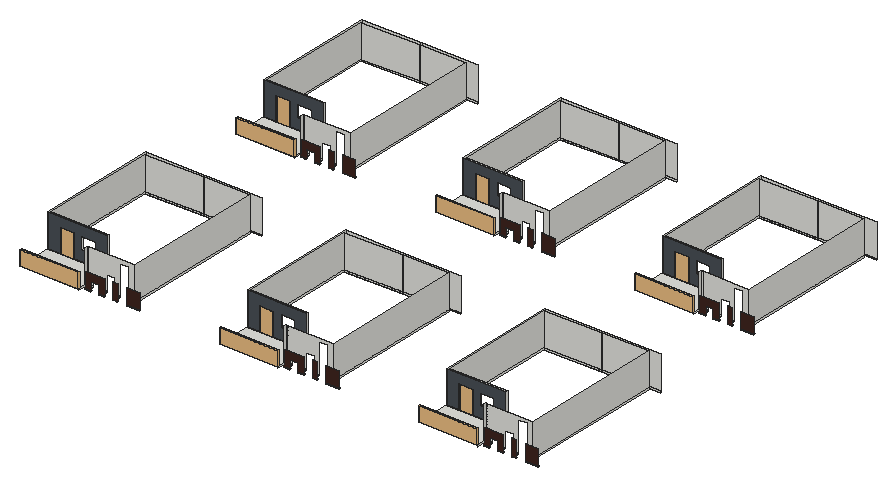
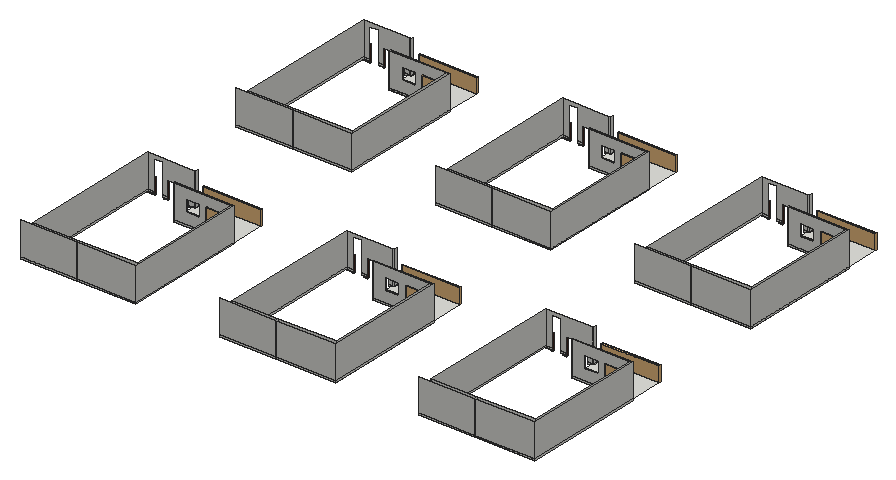
# SketchUp Ruby script. Lengths in inches.
U = 1.inch
M = Sketchup.active_model
def pt(a) = Geom::Point3d.new(a.map { |v| v * U })
def face(e, loops, mat)
  f = e.add_face(loops[0].map { |a| pt(a) })
  loops[1..].each { |l| e.add_face(l.map { |a| pt(a) }).erase! }
  f.material = f.back_material = mat if mat
  f
end
# faces: each face lists its corners as indices into pts; further lists are holes
def faces(e, pts, list, mat = nil) = list.each { |f| face(e, (f[0].is_a?(Array) ? f : [f]).map { |l| l.map { |i| pts[i] } }, mat) }
# xy, xz, yz: faces in a plane at the given z, y or x. An outline is a flat list of corners, or four numbers for a rectangle; further outlines are holes
def ring(l) = l.size == 4 ? [[l[0], l[1]], [l[2], l[1]], [l[2], l[3]], [l[0], l[3]]] : l.each_slice(2).to_a
def flat(e, list, mat, &to3) = list.each { |f| face(e, (f[0].is_a?(Array) ? f : [f]).map { |l| ring(l).map { |u, v| to3.(u, v) } }, mat) }
def xy(e, z, list, mat = nil) = flat(e, list, mat) { |x, y| [x, y, z] }
def xz(e, y, list, mat = nil) = flat(e, list, mat) { |x, z| [x, y, z] }
def yz(e, x, list, mat = nil) = flat(e, list, mat) { |y, z| [x, y, z] }
def lines(e, pts, list) = list.each { |a, b| e.add_line(pt(pts[a]), pt(pts[b])) }
# prism: a flat outline (further loops are holes) pulled along v
def prism(e, loops, v, mat = nil)
  f = face(e, loops, mat); d = Geom::Vector3d.new(v.map { |x| x * U })
  f.pushpull(f.normal.samedirection?(d) ? d.length : -d.length)
end
def box(e, o, s, mat = nil) = prism(e, [[o, [o[0] + s[0], o[1], o[2]], [o[0] + s[0], o[1] + s[1], o[2]], [o[0], o[1] + s[1], o[2]]]], [0, 0, s[2]], mat)
def at(x, y, z, deg = 0) = Geom::Transformation.translation(pt([x, y, z])) * Geom::Transformation.rotation(ORIGIN, Z_AXIS, deg.degrees)
def axes(o, x, y, z) = Geom::Transformation.new([*x, 0, *y, 0, *z, 0, *pt(o).to_a, 1])
def part(name) = M.definitions.add(name)
# library, detail: a bought-in or finely detailed component or shape, given as its bounding box
def library(name, o, s) = part(name).tap { |d| box(d.entities, o, s) }
def detail(e, o, s) = box(e.add_group.entities, o, s)
def put(e, d, t, mat = nil) = e.add_instance(d, t).tap { |i| i.material = mat if mat }
def group(e, t, mat = nil) = e.add_group.tap { |g| g.transformation = t; g.material = mat if mat }.entities
root = M.entities
M.materials.add("[0043_SaddleBrown]").color = [63, 38, 31]
M.materials.add("[Formica Blue]").color = [73, 80, 86]
c1 = library("Glass Railing",[0,0,0],[139.5,4.76,42])
c2 = library("door (1)",[38.93,25.48,0],[40,9.94,82.68])
xy(root,243.96,[[348.1875,438.72,370.54,441.04],[399.16,438.72,419.76,441.04],[451.01,438.72,467.3,441.04],[1072.625,438.72,1094.98,441.04],[1123.6,438.72,1144.2,441.04],
  [1175.45,438.72,1191.74,441.04],[1797.0625,438.72,1819.41,441.04],[1848.04,438.72,1868.64,441.04],[1899.89,438.72,1916.17,441.04],[500.42,438.73,547.05,441.04],
  [1224.86,438.73,1271.49,441.04],[1949.3,438.73,1995.93,441.04],[348.1875,1419.07,370.54,1421.39],[399.16,1419.07,419.76,1421.39],[451.01,1419.07,467.3,1421.39],
  [1072.625,1419.07,1094.98,1421.39],[1123.6,1419.07,1144.2,1421.39],[1175.45,1419.07,1191.74,1421.39],[1797.0625,1419.07,1819.41,1421.39],[1848.04,1419.07,1868.64,1421.39],
  [1899.89,1419.07,1916.17,1421.39],[500.42,1419.08,547.05,1421.39],[1224.86,1419.08,1271.49,1421.39],[1949.3,1419.08,1995.93,1421.39]])
xy(root,245.59,[[451.01,438.72,467.3,441.04],[1175.45,438.72,1191.74,441.04],[1899.89,438.72,1916.17,441.04],[451.01,1419.07,467.3,1421.39],[1175.45,1419.07,1191.74,1421.39],
  [1899.89,1419.07,1916.17,1421.39]])
xy(root,246.18,[[399.16,438.72,419.76,441.04],[1123.6,438.72,1144.2,441.04],[1848.04,438.72,1868.64,441.04],[399.16,1419.07,419.76,1421.39],[1123.6,1419.07,1144.2,1421.39],
  [1848.04,1419.07,1868.64,1421.39]])
xy(root,246.28,[[500.42,438.73,547.05,441.04],[1224.86,438.73,1271.49,441.04],[1949.3,438.73,1995.93,441.04],[500.42,1419.08,547.05,1421.39],[1224.86,1419.08,1271.49,1421.39],
  [1949.3,1419.08,1995.93,1421.39]])
xy(root,246.4375,[[348.1875,438.72,370.54,441.04],[1072.625,438.72,1094.98,441.04],[1797.0625,438.72,1819.41,441.04],[348.1875,1419.07,370.54,1421.39],[1072.625,1419.07,1094.98,1421.39],
  [1797.0625,1419.07,1819.41,1421.39]])
xy(root,252.25,[[137.5,535.375,137.5,980.35,353.97,980.35,353.97,971.23,144.84,965.96,144.84,540.48,353.97,540.48,353.97,535.375],[861.9375,535.375,861.9375,980.35,1078.41,980.35,1078.41,971.23,869.28,965.96,869.28,540.48,1078.41,540.48,1078.41,535.375],[1586.375,535.375,1586.375,980.35,1802.84,980.35,1802.84,971.23,1593.72,965.96,1593.72,540.48,1802.84,540.48,1802.84,535.375],[137.5,1515.73,137.5,1960.7,353.97,1960.7,353.97,1951.58,144.84,1946.3125,144.84,1520.83,353.97,1520.83,353.97,1515.73],[861.9375,1515.73,861.9375,1960.7,1078.41,1960.7,1078.41,1951.58,869.28,1946.3125,869.28,1520.83,1078.41,1520.83,1078.41,1515.73],
  [1586.375,1515.73,1586.375,1960.7,1802.84,1960.7,1802.84,1951.58,1593.72,1946.3125,1593.72,1520.83,1802.84,1520.83,1802.84,1515.73]])
xy(root,258.25,[[137.5,412.04,348.1875,412.04,348.1875,447.84,353.97,447.84,353.97,535.375,137.5,535.375],[861.9375,412.04,1072.625,412.04,1072.625,447.84,1078.41,447.84,1078.41,535.375,861.9375,535.375],[1586.375,412.04,1797.0625,412.04,1797.0625,447.84,1802.84,447.84,1802.84,535.375,1586.375,535.375],[137.5,535.375,137.5,980.35,353.97,980.35,353.97,971.23,144.84,965.96,144.84,540.48,183.3,540.48,183.3,535.375],[183.3,535.375,231.3,540.48],
  [231.3,535.375,353.97,540.48],[861.9375,535.375,861.9375,980.35,1078.41,980.35,1078.41,971.23,869.28,965.96,869.28,540.48,907.74,540.48,907.74,535.375],[907.74,535.375,955.74,540.48],[955.74,535.375,1078.41,540.48],[1586.375,535.375,1586.375,980.35,1802.84,980.35,1802.84,971.23,1593.72,965.96,1593.72,540.48,1632.17,540.48,1632.17,535.375],
  [1632.17,535.375,1680.17,540.48],[1680.17,535.375,1802.84,540.48],[137.5,1392.39,348.1875,1392.39,348.1875,1428.19,353.97,1428.19,353.97,1515.73,137.5,1515.73],[861.9375,1392.39,1072.625,1392.39,1072.625,1428.19,1078.41,1428.19,1078.41,1515.73,861.9375,1515.73],[1586.375,1392.39,1797.0625,1392.39,1797.0625,1428.19,1802.84,1428.19,1802.84,1515.73,1586.375,1515.73],
  [137.5,1515.73,137.5,1960.7,353.97,1960.7,353.97,1951.58,144.84,1946.3125,144.84,1520.83,183.3,1520.83,183.3,1515.73],[183.3,1515.73,231.3,1520.83],[231.3,1515.73,353.97,1520.83],[861.9375,1515.73,861.9375,1960.7,1078.41,1960.7,1078.41,1951.58,869.28,1946.3125,869.28,1520.83,907.74,1520.83,907.74,1515.73],[907.74,1515.73,955.74,1520.83],
  [955.74,1515.73,1078.41,1520.83],[1586.375,1515.73,1586.375,1960.7,1802.84,1960.7,1802.84,1951.58,1593.72,1946.3125,1593.72,1520.83,1632.17,1520.83,1632.17,1515.73],[1632.17,1515.73,1680.17,1520.83],[1680.17,1515.73,1802.84,1520.83]])
xy(root,275.89,[[370.54,438.72,399.16,447.84],[1094.98,438.72,1123.6,447.84],[1819.41,438.72,1848.04,447.84],[370.54,1419.07,399.16,1428.19],[1094.98,1419.07,1123.6,1428.19],
  [1819.41,1419.07,1848.04,1428.19]])
xz(root,438.72,[[451.01,245.59,467.3,303],[1175.45,245.59,1191.74,303],[1899.89,245.59,1916.17,303],[399.16,246.18,419.76,246.18,419.76,303,348.1875,303,348.1875,246.4375,370.54,246.4375,370.54,275.89,399.16,275.89],[1123.6,246.18,1144.2,246.18,1144.2,303,1072.625,303,1072.625,246.4375,1094.98,246.4375,1094.98,275.89,1123.6,275.89],
  [1848.04,246.18,1868.64,246.18,1868.64,303,1797.0625,303,1797.0625,246.4375,1819.41,246.4375,1819.41,275.89,1848.04,275.89]],"[0043_SaddleBrown]")
xz(root,438.73,[[500.42,246.28,547.05,303],[1224.86,246.28,1271.49,303],[1949.3,246.28,1995.93,303]],"[0043_SaddleBrown]")
xz(root,441.04,[[348.1875,243.96,370.54,246.4375],[399.16,243.96,419.76,246.18],[451.01,243.96,467.3,245.59],[500.42,243.96,547.05,246.28],[1072.625,243.96,1094.98,246.4375],
  [1123.6,243.96,1144.2,246.18],[1175.45,243.96,1191.74,245.59],[1224.86,243.96,1271.49,246.28],[1797.0625,243.96,1819.41,246.4375],[1848.04,243.96,1868.64,246.18],
  [1899.89,243.96,1916.17,245.59],[1949.3,243.96,1995.93,246.28]],"[0043_SaddleBrown]")
xz(root,447.84,[[348.1875,252.25,353.97,258.25],[353.97,252.25,370.54,258.25],[399.16,252.25,419.76,258.25],[451.01,252.25,467.3,258.25],[500.42,252.25,521.63,258.25],
  [1072.625,252.25,1078.41,258.25],[1078.41,252.25,1094.98,258.25],[1123.6,252.25,1144.2,258.25],[1175.45,252.25,1191.74,258.25],[1224.86,252.25,1246.07,258.25],
  [1797.0625,252.25,1802.84,258.25],[1802.84,252.25,1819.41,258.25],[1848.04,252.25,1868.64,258.25],[1899.89,252.25,1916.17,258.25],[1949.3,252.25,1970.51,258.25],
  [348.1875,258.25,353.97,378.25],[353.97,258.25,353.97,378.25,521.63,378.25,521.63,258.25,500.42,258.25,500.42,365.23,467.3,365.23,467.3,258.25,451.01,258.25,451.01,312.4,419.76,312.4,419.76,258.25,399.16,258.25,399.16,275.89,370.54,275.89,370.54,258.25],[1072.625,258.25,1078.41,378.25],[1078.41,258.25,1078.41,378.25,1246.07,378.25,1246.07,258.25,1224.86,258.25,1224.86,365.23,1191.74,365.23,1191.74,258.25,1175.45,258.25,1175.45,312.4,1144.2,312.4,1144.2,258.25,1123.6,258.25,1123.6,275.89,1094.98,275.89,1094.98,258.25],[1797.0625,258.25,1802.84,378.25],
  [1802.84,258.25,1802.84,378.25,1970.51,378.25,1970.51,258.25,1949.3,258.25,1949.3,365.23,1916.17,365.23,1916.17,258.25,1899.89,258.25,1899.89,312.4,1868.64,312.4,1868.64,258.25,1848.04,258.25,1848.04,275.89,1819.41,275.89,1819.41,258.25]])
xz(root,535.375,[[137.5,252.25,353.97,258.25],[861.9375,252.25,1078.41,258.25],[1586.375,252.25,1802.84,258.25]])
xz(root,535.375,[[[137.5,258.25,183.3,258.25,183.3,342.25,231.3,342.25,231.3,258.25,353.97,258.25,353.97,378.25,137.5,378.25],[258.09,298.0625,309.84,342.25]],[[861.9375,258.25,907.74,258.25,907.74,342.25,955.74,342.25,955.74,258.25,1078.41,258.25,1078.41,378.25,861.9375,378.25],[982.53,298.0625,1034.28,342.25]],[[1586.375,258.25,1632.17,258.25,1632.17,342.25,1680.17,342.25,1680.17,258.25,1802.84,258.25,1802.84,378.25,1586.375,378.25],[1706.96,298.0625,1758.71,342.25]]],"[Formica Blue]")
xz(root,540.48,[[144.84,252.25,353.97,258.25],[869.28,252.25,1078.41,258.25],[1593.72,252.25,1802.84,258.25],[[144.84,258.25,144.84,378.25,353.97,378.25,353.97,258.25,231.3,258.25,231.3,342.25,183.3,342.25,183.3,258.25],[258.09,298.0625,309.84,342.25]],[[869.28,258.25,869.28,378.25,1078.41,378.25,1078.41,258.25,955.74,258.25,955.74,342.25,907.74,342.25,907.74,258.25],[982.53,298.0625,1034.28,342.25]],
  [[1593.72,258.25,1593.72,378.25,1802.84,378.25,1802.84,258.25,1680.17,258.25,1680.17,342.25,1632.17,342.25,1632.17,258.25],[1706.96,298.0625,1758.71,342.25]]])
xz(root,971.23,[[353.97,252.25,521.63,258.25],[1078.41,252.25,1246.07,258.25],[1802.84,252.25,1970.51,258.25],[353.97,258.25,521.63,378.25],[1078.41,258.25,1246.07,378.25],
  [1802.84,258.25,1970.51,378.25]])
xz(root,980.35,[[137.5,252.25,353.97,258.25],[353.97,252.25,558.625,258.25],[861.9375,252.25,1078.41,258.25],[1078.41,252.25,1283.0625,258.25],[1586.375,252.25,1802.84,258.25],
  [1802.84,252.25,2007.5,258.25],[137.5,258.25,353.97,378.25],[353.97,258.25,558.625,378.25],[861.9375,258.25,1078.41,378.25],[1078.41,258.25,1283.0625,378.25],
  [1586.375,258.25,1802.84,378.25],[1802.84,258.25,2007.5,378.25]])
xz(root,1419.07,[[451.01,245.59,467.3,303],[1175.45,245.59,1191.74,303],[1899.89,245.59,1916.17,303],[399.16,246.18,419.76,246.18,419.76,303,348.1875,303,348.1875,246.4375,370.54,246.4375,370.54,275.89,399.16,275.89],[1123.6,246.18,1144.2,246.18,1144.2,303,1072.625,303,1072.625,246.4375,1094.98,246.4375,1094.98,275.89,1123.6,275.89],
  [1848.04,246.18,1868.64,246.18,1868.64,303,1797.0625,303,1797.0625,246.4375,1819.41,246.4375,1819.41,275.89,1848.04,275.89]],"[0043_SaddleBrown]")
xz(root,1419.08,[[500.42,246.28,547.05,303],[1224.86,246.28,1271.49,303],[1949.3,246.28,1995.93,303]],"[0043_SaddleBrown]")
xz(root,1421.39,[[348.1875,243.96,370.54,246.4375],[399.16,243.96,419.76,246.18],[451.01,243.96,467.3,245.59],[500.42,243.96,547.05,246.28],[1072.625,243.96,1094.98,246.4375],
  [1123.6,243.96,1144.2,246.18],[1175.45,243.96,1191.74,245.59],[1224.86,243.96,1271.49,246.28],[1797.0625,243.96,1819.41,246.4375],[1848.04,243.96,1868.64,246.18],
  [1899.89,243.96,1916.17,245.59],[1949.3,243.96,1995.93,246.28]],"[0043_SaddleBrown]")
xz(root,1428.19,[[348.1875,252.25,353.97,258.25],[353.97,252.25,370.54,258.25],[399.16,252.25,419.76,258.25],[451.01,252.25,467.3,258.25],[500.42,252.25,521.63,258.25],
  [1072.625,252.25,1078.41,258.25],[1078.41,252.25,1094.98,258.25],[1123.6,252.25,1144.2,258.25],[1175.45,252.25,1191.74,258.25],[1224.86,252.25,1246.07,258.25],
  [1797.0625,252.25,1802.84,258.25],[1802.84,252.25,1819.41,258.25],[1848.04,252.25,1868.64,258.25],[1899.89,252.25,1916.17,258.25],[1949.3,252.25,1970.51,258.25],
  [348.1875,258.25,353.97,378.25],[353.97,258.25,353.97,378.25,521.63,378.25,521.63,258.25,500.42,258.25,500.42,365.23,467.3,365.23,467.3,258.25,451.01,258.25,451.01,312.4,419.76,312.4,419.76,258.25,399.16,258.25,399.16,275.89,370.54,275.89,370.54,258.25],[1072.625,258.25,1078.41,378.25],[1078.41,258.25,1078.41,378.25,1246.07,378.25,1246.07,258.25,1224.86,258.25,1224.86,365.23,1191.74,365.23,1191.74,258.25,1175.45,258.25,1175.45,312.4,1144.2,312.4,1144.2,258.25,1123.6,258.25,1123.6,275.89,1094.98,275.89,1094.98,258.25],[1797.0625,258.25,1802.84,378.25],
  [1802.84,258.25,1802.84,378.25,1970.51,378.25,1970.51,258.25,1949.3,258.25,1949.3,365.23,1916.17,365.23,1916.17,258.25,1899.89,258.25,1899.89,312.4,1868.64,312.4,1868.64,258.25,1848.04,258.25,1848.04,275.89,1819.41,275.89,1819.41,258.25]])
xz(root,1515.73,[[137.5,252.25,353.97,258.25],[861.9375,252.25,1078.41,258.25],[1586.375,252.25,1802.84,258.25]])
xz(root,1515.73,[[[137.5,258.25,183.3,258.25,183.3,342.25,231.3,342.25,231.3,258.25,353.97,258.25,353.97,378.25,137.5,378.25],[258.09,298.0625,309.84,342.25]],[[861.9375,258.25,907.74,258.25,907.74,342.25,955.74,342.25,955.74,258.25,1078.41,258.25,1078.41,378.25,861.9375,378.25],[982.53,298.0625,1034.28,342.25]],[[1586.375,258.25,1632.17,258.25,1632.17,342.25,1680.17,342.25,1680.17,258.25,1802.84,258.25,1802.84,378.25,1586.375,378.25],[1706.96,298.0625,1758.71,342.25]]],"[Formica Blue]")
xz(root,1520.83,[[144.84,252.25,353.97,258.25],[869.28,252.25,1078.41,258.25],[1593.72,252.25,1802.84,258.25],[[144.84,258.25,144.84,378.25,353.97,378.25,353.97,258.25,231.3,258.25,231.3,342.25,183.3,342.25,183.3,258.25],[258.09,298.0625,309.84,342.25]],[[869.28,258.25,869.28,378.25,1078.41,378.25,1078.41,258.25,955.74,258.25,955.74,342.25,907.74,342.25,907.74,258.25],[982.53,298.0625,1034.28,342.25]],
  [[1593.72,258.25,1593.72,378.25,1802.84,378.25,1802.84,258.25,1680.17,258.25,1680.17,342.25,1632.17,342.25,1632.17,258.25],[1706.96,298.0625,1758.71,342.25]]])
xz(root,1951.58,[[353.97,252.25,521.63,258.25],[1078.41,252.25,1246.07,258.25],[1802.84,252.25,1970.51,258.25],[353.97,258.25,521.63,378.25],[1078.41,258.25,1246.07,378.25],
  [1802.84,258.25,1970.51,378.25]])
xz(root,1960.7,[[137.5,252.25,353.97,258.25],[353.97,252.25,558.625,258.25],[861.9375,252.25,1078.41,258.25],[1078.41,252.25,1283.0625,258.25],[1586.375,252.25,1802.84,258.25],
  [1802.84,252.25,2007.5,258.25],[137.5,258.25,353.97,378.25],[353.97,258.25,558.625,378.25],[861.9375,258.25,1078.41,378.25],[1078.41,258.25,1283.0625,378.25],
  [1586.375,258.25,1802.84,378.25],[1802.84,258.25,2007.5,378.25]])
yz(root,137.5,[[535.375,252.25,980.35,258.25],[1515.73,252.25,1960.7,258.25],[535.375,258.25,980.35,378.25],[1515.73,258.25,1960.7,378.25]])
yz(root,144.84,[[540.48,252.25,965.96,258.25],[1520.83,252.25,1946.3125,258.25],[540.48,258.25,965.96,378.25],[1520.83,258.25,1946.3125,378.25]])
yz(root,183.3,[[535.375,258.25,540.48,342.25],[1515.73,258.25,1520.83,342.25]])
yz(root,231.3,[[535.375,258.25,540.48,342.25],[1515.73,258.25,1520.83,342.25]])
yz(root,348.1875,[[412.04,252.25,438.72,258.25],[438.72,252.25,447.84,258.25],[1392.39,252.25,1419.07,258.25],[1419.07,252.25,1428.19,258.25],[438.72,258.25,438.72,303,441.04,303,441.04,306.15,438.72,306.15,438.72,354.05,441.04,354.05,441.04,355.72,438.72,355.72,438.72,378.25,447.84,378.25,447.84,258.25],
  [1419.07,258.25,1419.07,303,1421.39,303,1421.39,306.15,1419.07,306.15,1419.07,354.05,1421.39,354.05,1421.39,355.72,1419.07,355.72,1419.07,378.25,1428.19,378.25,1428.19,258.25]])
yz(root,353.97,[[535.375,252.25,540.48,258.25],[971.23,252.25,980.35,258.25],[1515.73,252.25,1520.83,258.25],[1951.58,252.25,1960.7,258.25],[535.375,258.25,540.48,378.25],
  [971.23,258.25,980.35,378.25],[1515.73,258.25,1520.83,378.25],[1951.58,258.25,1960.7,378.25]])
yz(root,521.63,[[447.84,252.25,971.23,258.25],[1428.19,252.25,1951.58,258.25],[447.84,258.25,971.23,378.25],[1428.19,258.25,1951.58,378.25]])
yz(root,861.9375,[[535.375,252.25,980.35,258.25],[1515.73,252.25,1960.7,258.25],[535.375,258.25,980.35,378.25],[1515.73,258.25,1960.7,378.25]])
yz(root,869.28,[[540.48,252.25,965.96,258.25],[1520.83,252.25,1946.3125,258.25],[540.48,258.25,965.96,378.25],[1520.83,258.25,1946.3125,378.25]])
yz(root,907.74,[[535.375,258.25,540.48,342.25],[1515.73,258.25,1520.83,342.25]])
yz(root,955.74,[[535.375,258.25,540.48,342.25],[1515.73,258.25,1520.83,342.25]])
yz(root,1072.625,[[412.04,252.25,438.72,258.25],[438.72,252.25,447.84,258.25],[1392.39,252.25,1419.07,258.25],[1419.07,252.25,1428.19,258.25],[438.72,258.25,438.72,303,441.04,303,441.04,306.15,438.72,306.15,438.72,354.05,441.04,354.05,441.04,355.72,438.72,355.72,438.72,378.25,447.84,378.25,447.84,258.25],
  [1419.07,258.25,1419.07,303,1421.39,303,1421.39,306.15,1419.07,306.15,1419.07,354.05,1421.39,354.05,1421.39,355.72,1419.07,355.72,1419.07,378.25,1428.19,378.25,1428.19,258.25]])
yz(root,1078.41,[[535.375,252.25,540.48,258.25],[971.23,252.25,980.35,258.25],[1515.73,252.25,1520.83,258.25],[1951.58,252.25,1960.7,258.25],[535.375,258.25,540.48,378.25],
  [971.23,258.25,980.35,378.25],[1515.73,258.25,1520.83,378.25],[1951.58,258.25,1960.7,378.25]])
yz(root,1246.07,[[447.84,252.25,971.23,258.25],[1428.19,252.25,1951.58,258.25],[447.84,258.25,971.23,378.25],[1428.19,258.25,1951.58,378.25]])
yz(root,1586.375,[[535.375,252.25,980.35,258.25],[1515.73,252.25,1960.7,258.25],[535.375,258.25,980.35,378.25],[1515.73,258.25,1960.7,378.25]])
yz(root,1593.72,[[540.48,252.25,965.96,258.25],[1520.83,252.25,1946.3125,258.25],[540.48,258.25,965.96,378.25],[1520.83,258.25,1946.3125,378.25]])
yz(root,1632.17,[[535.375,258.25,540.48,342.25],[1515.73,258.25,1520.83,342.25]])
yz(root,1680.17,[[535.375,258.25,540.48,342.25],[1515.73,258.25,1520.83,342.25]])
yz(root,1797.0625,[[412.04,252.25,438.72,258.25],[438.72,252.25,447.84,258.25],[1392.39,252.25,1419.07,258.25],[1419.07,252.25,1428.19,258.25],[438.72,258.25,438.72,303,441.04,303,441.04,306.15,438.72,306.15,438.72,354.05,441.04,354.05,441.04,355.72,438.72,355.72,438.72,378.25,447.84,378.25,447.84,258.25],
  [1419.07,258.25,1419.07,303,1421.39,303,1421.39,306.15,1419.07,306.15,1419.07,354.05,1421.39,354.05,1421.39,355.72,1419.07,355.72,1419.07,378.25,1428.19,378.25,1428.19,258.25]])
yz(root,1802.84,[[535.375,252.25,540.48,258.25],[971.23,252.25,980.35,258.25],[1515.73,252.25,1520.83,258.25],[1951.58,252.25,1960.7,258.25],[535.375,258.25,540.48,378.25],
  [971.23,258.25,980.35,378.25],[1515.73,258.25,1520.83,378.25],[1951.58,258.25,1960.7,378.25]])
yz(root,1970.51,[[447.84,252.25,971.23,258.25],[1428.19,252.25,1951.58,258.25],[447.84,258.25,971.23,378.25],[1428.19,258.25,1951.58,378.25]])
p = [[144.84,965.96,252.25],[353.97,971.23,252.25],[353.97,971.23,258.25],[144.84,965.96,258.25],[869.28,965.96,252.25],[1078.41,971.23,252.25],
  [1078.41,971.23,258.25],[869.28,965.96,258.25],[1593.72,965.96,252.25],[1802.84,971.23,252.25],[1802.84,971.23,258.25],[1593.72,965.96,258.25],
  [144.84,1946.3125,252.25],[353.97,1951.58,252.25],[353.97,1951.58,258.25],[144.84,1946.3125,258.25],[869.28,1946.3125,252.25],[1078.41,1951.58,252.25],
  [1078.41,1951.58,258.25],[869.28,1946.3125,258.25],[1593.72,1946.3125,252.25],[1802.84,1951.58,252.25],[1802.84,1951.58,258.25],[1593.72,1946.3125,258.25],
  [353.97,971.23,378.25],[144.84,965.96,378.25],[1078.41,971.23,378.25],[869.28,965.96,378.25],[1802.84,971.23,378.25],[1593.72,965.96,378.25],
  [353.97,1951.58,378.25],[144.84,1946.3125,378.25],[1078.41,1951.58,378.25],[869.28,1946.3125,378.25],[1802.84,1951.58,378.25],[1593.72,1946.3125,378.25],
  [1078.41,447.84,252.25],[1078.41,438.72,252.25],[1078.41,447.84,258.25],[1078.41,438.72,258.25],[1802.84,447.84,252.25],[1802.84,438.72,252.25],
  [1802.84,447.84,258.25],[1802.84,438.72,258.25],[353.97,447.84,258.25],[353.97,438.72,258.25],[353.97,447.84,252.25],[353.97,438.72,252.25],
  [1078.41,1428.19,258.25],[1078.41,1419.07,258.25],[1078.41,1428.19,252.25],[1078.41,1419.07,252.25],[1802.84,1428.19,252.25],[1802.84,1419.07,252.25],
  [1802.84,1428.19,258.25],[1802.84,1419.07,258.25],[353.97,1428.19,258.25],[353.97,1419.07,258.25],[353.97,1428.19,252.25],[353.97,1419.07,252.25]]
faces(root,p,[[0,1,2,3],[4,5,6,7],[8,9,10,11],[12,13,14,15],[16,17,18,19],[20,21,22,23],[3,2,24,25],[7,6,26,27],
  [11,10,28,29],[15,14,30,31],[19,18,32,33],[23,22,34,35]])
lines(root,p,[[36,37],[38,39],[40,41],[42,43],[44,45],[46,47],[48,49],[50,51],[52,53],[54,55],[56,57],[58,59]])
put(root,c1,axes([1586.375,1389.32,258.21],[1.51031,0,0],[0,1.27,0],[0,0,1.27]))
put(root,c1,axes([861.9375,1389.32,258.21],[1.51031,0,0],[0,1.27,0],[0,0,1.27]))
put(root,c1,axes([137.5,1389.32,258.21],[1.51031,0,0],[0,1.27,0],[0,0,1.27]))
put(root,c1,axes([861.9375,408.97,258.21],[1.51031,0,0],[0,1.27,0],[0,0,1.27]))
put(root,c1,axes([1586.375,408.97,258.21],[1.51031,0,0],[0,1.27,0],[0,0,1.27]))
put(root,c1,axes([137.5,408.97,258.21],[1.51031,0,0],[0,1.27,0],[0,0,1.27]))
put(root,c2,axes([133.81,1490.24,258.25],[1.2351,0,0],[0,1,0],[0,0,1.016]))
put(root,c2,axes([858.25,1490.24,258.25],[1.2351,0,0],[0,1,0],[0,0,1.016]))
put(root,c2,axes([1582.69,1490.24,258.25],[1.2351,0,0],[0,1,0],[0,0,1.016]))
put(root,c2,axes([858.25,509.89,258.25],[1.2351,0,0],[0,1,0],[0,0,1.016]))
put(root,c2,axes([1582.69,509.89,258.25],[1.2351,0,0],[0,1,0],[0,0,1.016]))
put(root,c2,axes([133.81,509.89,258.25],[1.2351,0,0],[0,1,0],[0,0,1.016]))
